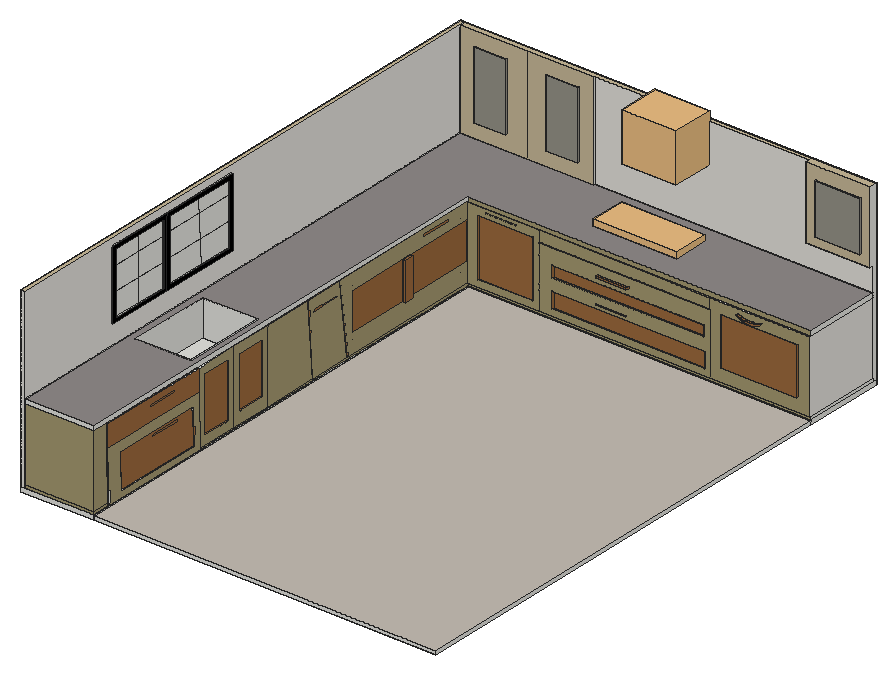
# SketchUp Ruby script. Lengths in inches.
U = 1.inch
M = Sketchup.active_model
def pt(a) = Geom::Point3d.new(a.map { |v| v * U })
def face(e, loops, mat)
  f = e.add_face(loops[0].map { |a| pt(a) })
  loops[1..].each { |l| e.add_face(l.map { |a| pt(a) }).erase! }
  f.material = f.back_material = mat if mat
  f
end
# faces: each face lists its corners as indices into pts; further lists are holes
def faces(e, pts, list, mat = nil) = list.each { |f| face(e, (f[0].is_a?(Array) ? f : [f]).map { |l| l.map { |i| pts[i] } }, mat) }
# xy, xz, yz: faces in a plane at the given z, y or x. An outline is a flat list of corners, or four numbers for a rectangle; further outlines are holes
def ring(l) = l.size == 4 ? [[l[0], l[1]], [l[2], l[1]], [l[2], l[3]], [l[0], l[3]]] : l.each_slice(2).to_a
def flat(e, list, mat, &to3) = list.each { |f| face(e, (f[0].is_a?(Array) ? f : [f]).map { |l| ring(l).map { |u, v| to3.(u, v) } }, mat) }
def xy(e, z, list, mat = nil) = flat(e, list, mat) { |x, y| [x, y, z] }
def xz(e, y, list, mat = nil) = flat(e, list, mat) { |x, z| [x, y, z] }
def yz(e, x, list, mat = nil) = flat(e, list, mat) { |y, z| [x, y, z] }
def lines(e, pts, list) = list.each { |a, b| e.add_line(pt(pts[a]), pt(pts[b])) }
# prism: a flat outline (further loops are holes) pulled along v
def prism(e, loops, v, mat = nil)
  f = face(e, loops, mat); d = Geom::Vector3d.new(v.map { |x| x * U })
  f.pushpull(f.normal.samedirection?(d) ? d.length : -d.length)
end
def box(e, o, s, mat = nil) = prism(e, [[o, [o[0] + s[0], o[1], o[2]], [o[0] + s[0], o[1] + s[1], o[2]], [o[0], o[1] + s[1], o[2]]]], [0, 0, s[2]], mat)
def at(x, y, z, deg = 0) = Geom::Transformation.translation(pt([x, y, z])) * Geom::Transformation.rotation(ORIGIN, Z_AXIS, deg.degrees)
def axes(o, x, y, z) = Geom::Transformation.new([*x, 0, *y, 0, *z, 0, *pt(o).to_a, 1])
def part(name) = M.definitions.add(name)
# library, detail: a bought-in or finely detailed component or shape, given as its bounding box
def library(name, o, s) = part(name).tap { |d| box(d.entities, o, s) }
def detail(e, o, s) = box(e.add_group.entities, o, s)
def put(e, d, t, mat = nil) = e.add_instance(d, t).tap { |i| i.material = mat if mat }
def group(e, t, mat = nil) = e.add_group.tap { |g| g.transformation = t; g.material = mat if mat }.entities
root = M.entities
M.materials.add("[Color M09]").color = [0, 0, 0]
M.materials.add("[Field Rectangle Tile]").color = [196, 189, 179]
M.materials.add("[Formica Graystone]").color = [149, 146, 135]
M.materials.add("[Marble Carrara Gold Floor Tile]").color = [225, 223, 217]
M.materials.add("[Quartz Light Brown]").color = [199, 184, 152]
M.materials.add("[Stone Marble]").color = [143, 138, 136]
M.materials.add("[Wood Floor]").color = [155, 105, 61]
M.materials.add("[Wood Lumber ButtJoined]").color = [164, 152, 112]
c1 = library("CGP650SETSS",[0,0,0],[36,20.75,4.5])
c2 = library("PV977NSS_GEProfile",[-17.9375,-27.5625,-0.25],[35.95,27.64,32.08])
xy(root,0,[[0,0,0,365.375,276.25,365.375,276.25,311.14,48.625,311.14,48.625,0],[48.625,0,276.25,311.14]])
xy(root,2.4,[[48.625,0,276.25,311.14]],"[Field Rectangle Tile]")
xy(root,3,[[0,0,3,365.375],[3,0,3,362.375,276.25,362.375,276.25,311.14,48.625,311.14,48.625,0],[3,362.375,276.25,365.375]])
xy(root,5,[[3,0,3,362.375,276.25,362.375,276.25,311.14,48.625,311.14,48.625,0],[48.625,85.77,49.625,114.5],[48.625,114.5,49.625,143.24],[48.625,143.24,48.625,310.14,48.63,310.14,49.23,210.02,48.625,210.01,48.63,208.96,49.23,208.96,49.4,181.37,48.625,181.36,48.63,180.08,49.41,180.09,49.625,143.24],[48.625,310.14,48.625,311.14,48.63,310.14],
  [48.63,310.14,48.625,311.14,96,311.14,96,310.14],[96,310.14,210.05,311.14],[210.05,310.14,276.25,311.14]])
xy(root,9.28,[[105.11,310.14,206.3,311.14]],"[Wood Floor]")
xy(root,9.41,[[55.64,310.14,92.32,311.14]],"[Wood Floor]")
xy(root,11.1,[[48.625,90.01,49.625,110.7]],"[Wood Floor]")
xy(root,12.77,[[48.625,119.14,49.625,139.2]],"[Wood Floor]")
xy(root,14.16,[[217.67,309.14,268.43,310.14]],"[Wood Floor]")
xy(root,17.5625,[[48.2,213.88,49.2,213.88,48.95,256.07,47.95,256.07],[47.95,256.07,48.95,256.07,48.91,262.51,47.91,262.51],[47.91,262.51,48.91,262.51,48.625,311.14,47.625,311.13]])
xy(root,17.5625,[[48.95,256.07,48.91,262.51,50.91,262.52,50.95,256.08]],"[Wood Floor]")
xy(root,19.85,[[105.11,310.14,206.3,311.14]])
xy(root,28.14,[[105.21,310.14,206.08,311.14]],"[Wood Floor]")
xy(root,32,[[7.71,85.84,44.64,141.53]])
xy(root,35.58,[[105.21,310.14,206.08,311.14]])
xy(root,39.34,[[135.71,308.14,155.96,310.14]])
xy(root,40.4,[[135.71,308.14,155.96,310.14]],"[Wood Floor]")
xy(root,42.88,[[48.2,213.88,47.95,256.07,48.95,256.07,49.2,213.88],[47.95,256.07,47.91,262.51,48.91,262.51,48.95,256.07],[47.91,262.51,47.625,311.13,48.625,311.14,48.91,262.51]])
xy(root,42.88,[[48.95,256.07,50.95,256.08,50.91,262.52,48.91,262.51]],"[Wood Floor]")
xy(root,45.53,[[217.67,309.14,268.43,310.14]],"[Wood Floor]")
xy(root,46.96,[[48.625,119.14,49.625,139.2]],"[Wood Floor]")
xy(root,47.72,[[55.64,310.14,92.32,311.14]])
xy(root,47.85,[[48.625,90.01,49.625,110.7]],"[Wood Floor]")
xy(root,53,[[48.625,85.77,49.625,114.5],[48.625,114.5,49.625,143.24],[48.625,143.24,49.625,143.24,49.43,176.36,48.65,176.35,48.65,177.34,49.42,177.35,49.27,202.84,48.67,202.83,48.66,203.75,49.26,203.75,48.63,310.14,48.625,310.14],[48.625,310.14,48.63,310.14,48.625,311.14]])
xy(root,53,[[210.05,310.14,276.25,311.14]],"[Marble Carrara Gold Floor Tile]")
xy(root,53,[[48.63,310.14,96,310.14,96,311.14,48.625,311.14],[96,310.14,210.05,311.14]],"[Wood Lumber ButtJoined]")
xy(root,56,[[3,361.375,47.37,362.375],[47.37,361.375,91.74,362.375]])
xy(root,56,[[[3,0,48.625,0,48.625,311.14,276.25,311.14,276.25,362.375,91.74,362.375,91.74,361.375,3,361.375],[7.71,85.84,44.64,141.53]]],"[Stone Marble]")
xy(root,65.88,[[13.14,360.375,34.2,361.375]])
xy(root,65.88,[[60.64,360.375,81.7,361.375]],"[Formica Graystone]")
xy(root,69.45,[[3,72.13,4,116.73],[3,116.73,4,171.32]])
xy(root,71.58,[[3,74.26,4,94.43],[3,94.43,4,114.6]],"[Color M09]")
xy(root,71.82,[[3,119.1,4,146.39],[3,146.39,4,168.95]],"[Color M09]")
xy(root,72.01,[[233.56,360.375,276.25,362.375]],"[Quartz Light Brown]")
xy(root,78.16,[[240.1875,359.375,270.125,360.375]],"[Formica Graystone]")
xy(root,110.69,[[13.14,360.375,34.2,361.375],[60.64,360.375,81.7,361.375]],"[Formica Graystone]")
xy(root,111.41,[[240.1875,359.375,270.125,360.375]],"[Formica Graystone]")
xy(root,112.89,[[3,119.1,4,144.03],[3,144.03,4,168.95]])
xy(root,113.13,[[3,74.26,4,94.43],[3,94.43,4,114.6]])
xy(root,115.26,[[3,72.13,4,116.73],[3,116.73,4,171.32]],"[Color M09]")
xy(root,120,[[0,0,3,365.375],[233.56,360.375,276.25,360.375,276.25,365.375,3,365.375,3,361.375,91.74,361.375,91.74,362.375,233.56,362.375]],"[Quartz Light Brown]")
xz(root,0,[[0,0,48.625,3],[48.625,0,276.25,2.4],[3,53,48.625,56]])
xz(root,0,[[0,3,3,120]],"[Marble Carrara Gold Floor Tile]")
xz(root,0,[[3,3,48.625,5],[3,5,48.625,53]],"[Wood Lumber ButtJoined]")
xz(root,10.64,[[49.625,5,50.625,5.02,49.92,38.78,48.92,38.75],[48.92,38.75,49.92,38.78,49.625,53.02,48.625,53]])
xz(root,20.09,[[49.55,8.65,49.05,32.52,50.05,32.54,50.55,8.67]],"[Wood Floor]")
xz(root,72.13,[[3,69.45,4,115.26]],"[Color M09]")
xz(root,74.26,[[3,71.58,4,87.12],[3,87.12,4,102.65],[3,102.65,4,113.13]],"[Color M09]")
xz(root,81.46,[[49.55,8.65,50.55,8.67,50.05,32.54,49.05,32.52]],"[Wood Floor]")
xz(root,85.77,[[48.625,5,49.625,5,48.92,38.75,48.625,53],[49.625,5,49.625,38.77,48.92,38.75],[49.625,5,49.625,38.77,49.92,38.78,50.625,5.02],[48.92,38.75,49.625,38.77,49.625,53,48.625,53],[49.625,38.77,49.625,53,49.92,38.78],
  [48.625,53,49.625,53.02,49.625,53]])
xz(root,85.84,[[7.71,32,44.64,56]])
xz(root,90.01,[[48.625,11.1,49.625,47.85]],"[Wood Floor]")
xz(root,110.7,[[48.625,11.1,49.625,47.85]],"[Wood Floor]")
xz(root,114.6,[[3,71.58,4,87.12],[3,87.12,4,102.65],[3,102.65,4,113.13]],"[Color M09]")
xz(root,116.73,[[3,69.45,4,115.26]])
xz(root,119.1,[[3,71.82,4,87.55],[3,87.55,4,103.27],[3,103.27,4,112.89]],"[Color M09]")
xz(root,119.14,[[48.625,12.77,49.625,46.96]],"[Wood Floor]")
xz(root,139.2,[[48.625,12.77,49.625,46.96]],"[Wood Floor]")
xz(root,141.53,[[7.71,32,44.64,56]])
xz(root,143.24,[[48.625,5,49.625,53]])
xz(root,168.95,[[3,71.82,4,87.55],[3,87.55,4,103.27],[3,103.27,4,112.89]],"[Color M09]")
xz(root,171.32,[[3,69.45,4,115.26]],"[Color M09]")
xz(root,213.88,[[48.2,17.5625,49.2,42.88]])
xz(root,256.07,[[47.95,17.5625,48.95,42.88]],"[Wood Floor]")
xz(root,262.51,[[47.91,17.5625,48.91,42.88]])
xz(root,308.14,[[135.71,23.15,155.96,24.21],[135.71,39.34,155.96,40.4],[237.21,47.2,238.71,47.28,240.19,47.52,241.65,47.91,243.05,48.46,244.39,49.15,245.64,49.98,244.29,49.48,242.91,49.08,241.5,48.76,240.08,48.53,238.64,48.4,237.21,48.35,235.77,48.4,234.33,48.53,232.91,48.76,231.5,49.08,230.12,49.48,228.77,49.98,230.02,49.15,231.36,48.46,232.76,47.91,234.22,47.52,235.7,47.28]],"[Wood Floor]")
xz(root,309.14,[[217.67,14.16,268.43,45.53]],"[Wood Floor]")
xz(root,310.14,[[96,45.7,210.05,46.01],[60.76,50.07,81.01,51.14]],"[Wood Floor]")
xz(root,310.14,[[[48.625,5,96,53],[55.64,9.41,92.32,47.72],[60.76,50.07,81.01,51.14]],[[96,5,210.05,45.7],[105.11,9.28,206.3,19.85],[105.21,28.14,206.08,35.58],[135.71,39.34,155.96,40.4]],[[210.05,5,276.25,53],[217.67,14.16,268.43,45.53],[237.21,47.2,235.7,47.28,234.22,47.52,232.76,47.91,231.36,48.46,230.02,49.15,228.77,49.98,230.12,49.48,231.5,49.08,232.91,48.76,234.33,48.53,235.77,48.4,237.21,48.35,238.64,48.4,240.08,48.53,241.5,48.76,242.91,49.08,244.29,49.48,245.64,49.98,244.39,49.15,243.05,48.46,241.65,47.91,240.19,47.52,238.71,47.28]],[96,46.01,210.05,53]],"[Wood Lumber ButtJoined]")
xz(root,311.14,[[48.625,0,276.25,2.4],[48.625,2.4,276.25,3]])
xz(root,311.14,[[105.11,9.28,206.3,19.85],[55.64,9.41,92.32,47.72],[105.21,28.14,206.08,35.58]],"[Wood Floor]")
xz(root,311.14,[[48.625,3,276.25,5],[48.625,53,276.25,56]],"[Wood Lumber ButtJoined]")
xz(root,359.375,[[240.1875,78.16,270.125,111.41]],"[Formica Graystone]")
xz(root,360.375,[[13.14,65.88,34.2,110.69],[60.64,65.88,81.7,110.69]],"[Formica Graystone]")
xz(root,360.375,[[[233.56,72.01,276.25,120],[240.1875,78.16,270.125,111.41]]],"[Quartz Light Brown]")
xz(root,361.375,[[[3,56,47.37,120],[13.14,65.88,34.2,110.69]],[[47.37,56,91.74,120],[60.64,65.88,81.7,110.69]]],"[Quartz Light Brown]")
xz(root,362.375,[[3,3,276.25,5],[3,5,276.25,53],[3,53,276.25,56]])
xz(root,362.375,[[91.74,56,276.25,56,276.25,72.01,233.56,72.01,233.56,120,91.74,120]],"[Marble Carrara Gold Floor Tile]")
xz(root,365.375,[[0,0,276.25,3],[0,3,3,120],[3,3,276.25,120]])
yz(root,0,[[0,0,365.375,3],[0,3,365.375,120]])
yz(root,3,[[0,3,362.375,5],[362.375,3,365.375,3,365.375,120,361.375,120,361.375,56,362.375,56],[0,5,362.375,53],[0,53,362.375,56],[[72.13,69.45,116.73,115.26],[74.26,71.58,114.6,113.13]],
  [[116.73,69.45,171.32,115.26],[119.1,71.82,168.95,112.89]]])
yz(root,3,[[[0,56,361.375,120],[72.13,69.45,171.32,115.26]]],"[Marble Carrara Gold Floor Tile]")
yz(root,4,[[[72.13,69.45,116.73,115.26],[74.26,71.58,114.6,113.13]],[[116.73,69.45,171.32,115.26],[119.1,71.82,168.95,112.89]]],"[Color M09]")
yz(root,7.71,[[85.84,32,141.53,56]])
yz(root,13.14,[[360.375,65.88,361.375,110.69]],"[Formica Graystone]")
yz(root,34.2,[[360.375,65.88,361.375,110.69]],"[Formica Graystone]")
yz(root,44.64,[[85.84,32,141.53,56]])
yz(root,48.625,[[0,0,311.14,2.4],[0,2.4,311.14,3],[310.14,5,311.14,17.5625],[310.14,17.5625,311.14,42.88],[310.14,42.88,311.14,53],
  [0,53,311.14,56]])
yz(root,48.625,[[143.24,5,310.14,53],[90.01,11.1,110.7,47.85],[119.14,12.77,139.2,46.96]],"[Wood Floor]")
yz(root,48.625,[[0,3,311.14,5],[0,5,85.77,53]],"[Wood Lumber ButtJoined]")
yz(root,49.625,[[[85.77,5,114.5,53],[90.01,11.1,110.7,47.85]],[[114.5,5,143.24,53],[119.14,12.77,139.2,46.96]]],"[Wood Lumber ButtJoined]")
yz(root,55.64,[[310.14,9.41,311.14,47.72]],"[Wood Floor]")
yz(root,60.64,[[360.375,65.88,361.375,110.69]],"[Formica Graystone]")
yz(root,81.7,[[360.375,65.88,361.375,110.69]],"[Formica Graystone]")
yz(root,91.74,[[361.375,56,362.375,120]])
yz(root,92.32,[[310.14,9.41,311.14,47.72]],"[Wood Floor]")
yz(root,105.11,[[310.14,9.28,311.14,19.85]],"[Wood Floor]")
yz(root,105.21,[[310.14,28.14,311.14,35.58]],"[Wood Floor]")
yz(root,135.71,[[308.14,39.34,310.14,40.4]],"[Wood Floor]")
yz(root,155.96,[[308.14,39.34,310.14,40.4]],"[Wood Floor]")
yz(root,206.08,[[310.14,28.14,311.14,35.58]],"[Wood Floor]")
yz(root,206.3,[[310.14,9.28,311.14,19.85]],"[Wood Floor]")
yz(root,217.67,[[309.14,14.16,310.14,45.53]],"[Wood Floor]")
yz(root,233.56,[[360.375,72.01,362.375,120]])
yz(root,240.1875,[[359.375,78.16,360.375,111.41]],"[Formica Graystone]")
yz(root,268.43,[[309.14,14.16,310.14,45.53]],"[Wood Floor]")
yz(root,270.125,[[359.375,78.16,360.375,111.41]],"[Formica Graystone]")
yz(root,276.25,[[0,0,311.14,2.4],[311.14,0,365.375,3],[311.14,3,362.375,5],[362.375,3,365.375,3,365.375,120,360.375,120,360.375,72.01,362.375,72.01],[311.14,53,362.375,56]])
yz(root,276.25,[[310.14,5,362.375,53]],"[Marble Carrara Gold Floor Tile]")
p = [[48.92,85.77,38.75],[49.625,85.77,5],[49.625,10.64,5],[48.92,10.64,38.75],[49.55,81.46,8.65],[49.05,81.46,32.52],
  [49.05,20.09,32.52],[49.55,20.09,8.65],[50.625,85.77,5.02],[50.625,10.64,5.02],[49.92,85.77,38.78],[49.92,10.64,38.78],
  [50.05,81.46,32.54],[50.55,81.46,8.67],[50.55,20.09,8.67],[50.05,20.09,32.54],[49.625,143.24,5],[49.41,180.09,5],
  [49.43,176.36,53],[49.625,143.24,53],[49.47,169.09,39.49],[49.47,169.09,38.43],[49.59,148.84,38.43],[49.59,148.84,39.49],
  [48.63,180.08,5],[48.625,181.36,5],[48.65,177.34,53],[48.65,176.35,53],[49.4,181.37,5],[49.42,177.35,53],
  [49.23,208.96,5],[49.27,202.84,53],[49.27,202.01,45.33],[49.27,202.01,44.26],[49.4,181.76,44.26],[49.4,181.76,45.33],
  [48.63,208.96,5],[48.625,210.01,5],[48.66,203.75,53],[48.67,202.83,53],[48.625,311.14,5],[48.625,311.14,17.5625],
  [48.91,262.51,17.5625],[48.95,256.07,17.5625],[49.2,213.88,17.5625],[49.2,213.88,42.88],[48.95,256.07,42.88],[48.91,262.51,42.88],
  [48.625,311.14,42.88],[48.625,311.14,53],[48.63,310.14,53],[49.26,203.75,53],[49.23,210.02,5],[48.63,310.14,5],
  [48.73,293.66,49.63],[48.73,293.66,48.57],[48.85,273.41,48.57],[48.85,273.41,49.63],[49.11,68.46,29.95],[49.13,68.46,28.89],
  [49.13,48.21,28.89],[49.11,48.21,29.95],[5.95,213.99,45.65],[5.95,213.99,13.83],[5.41,304.36,13.83],[5.41,304.36,45.65],
  [47.95,256.07,17.5625],[47.91,262.51,17.5625],[47.91,262.51,42.88],[47.95,256.07,42.88],[50.95,256.08,17.5625],[50.95,256.08,42.88],
  [50.91,262.52,17.5625],[50.91,262.52,42.88],[47.625,311.13,42.88],[47.625,311.13,17.5625],[48.625,10.64,53],[48.625,85.77,53],
  [49.625,85.77,38.77],[49.625,10.64,53.02],[49.625,85.77,53],[49.625,85.77,53.02],[49.72,65.33,48.42],[49.74,65.33,47.36],
  [49.74,45.08,47.36],[49.72,45.08,48.42],[235.7,310.14,47.28],[237.21,310.14,47.2],[237.21,308.14,47.2],[235.7,308.14,47.28],
  [238.71,310.14,47.28],[238.71,308.14,47.28],[234.22,310.14,47.52],[234.22,308.14,47.52],[240.19,310.14,47.52],[240.19,308.14,47.52],
  [232.76,310.14,47.91],[232.76,308.14,47.91],[241.65,310.14,47.91],[241.65,308.14,47.91],[231.36,310.14,48.46],[231.36,308.14,48.46],
  [243.05,310.14,48.46],[243.05,308.14,48.46],[235.77,310.14,48.4],[234.33,310.14,48.53],[234.33,308.14,48.53],[235.77,308.14,48.4],
  [237.21,310.14,48.35],[237.21,308.14,48.35],[238.64,310.14,48.4],[238.64,308.14,48.4],[240.08,310.14,48.53],[240.08,308.14,48.53],
  [230.02,310.14,49.15],[230.02,308.14,49.15],[232.91,310.14,48.76],[232.91,308.14,48.76],[241.5,310.14,48.76],[241.5,308.14,48.76],
  [244.39,310.14,49.15],[244.39,308.14,49.15],[231.5,310.14,49.08],[231.5,308.14,49.08],[242.91,310.14,49.08],[242.91,308.14,49.08],
  [228.77,310.14,49.98],[228.77,308.14,49.98],[230.12,310.14,49.48],[230.12,308.14,49.48],[244.29,310.14,49.48],[244.29,308.14,49.48],
  [245.64,310.14,49.98],[245.64,308.14,49.98],[347.17,609.45,0],[347.17,609.45,-0.8125],[49.2,214.25,13.83],[49.2,214.25,45.65],
  [48.66,304.62,13.83],[48.66,304.62,45.65],[3,94.43,111.375],[3,94.43,102.65],[3,94.43,113.13],[3,74.26,102.65],
  [3,94.43,87.12],[3,114.6,102.65],[3,74.26,87.12],[3,94.43,71.58],[3,114.6,87.12],[3,144.03,112.89],
  [3,144.58,103.27],[3,119.1,103.27],[3,145.49,87.55],[3,168.95,103.27],[3,119.1,87.55],[3,146.39,71.82],
  [3,168.95,87.55]]
faces(root,p,[[[0,1,2,3],[4,5,6,7]],[2,1,8,9],[62,63,64,65],[66,67,68,69],[43,46,47,42],[41,48,74,75],[3,76,77,0],[0,3,11,10,78],
  [86,87,88,89],[87,90,91,88],[92,86,89,93],[90,94,95,91],[96,92,93,97],[94,98,99,95],[100,96,97,101],[98,102,103,99],
  [114,100,101,115],[102,120,121,103],[126,114,115,127],[120,132,133,121],[77,76,79,81]])
faces(root,p,[[[8,10,11,9],[12,13,14,15]],[[16,17,18,19],[20,21,22,23]],[[28,30,31,29],[32,33,34,35]],[[40,41,42,43,44,45,46,47,48,49,50,51,52,53],[54,55,56,57]]],"[Wood Lumber ButtJoined]")
faces(root,p,[[24,25,26,27],[18,17,24,27],[28,29,26,25],[36,37,38,39],[31,30,36,39],[52,51,38,37],[[4,5,6,7],[58,59,60,61]],[4,7,14,13],
  [46,43,70,71],[71,70,72,73],[42,47,73,72],[61,60,59,58],[6,5,12,15],[23,22,21,20],[[79,11,10,80,81],[82,83,84,85]],[35,34,33,32],
  [85,84,83,82],[104,105,106,107],[108,104,107,109],[110,108,109,111],[112,110,111,113],[105,116,117,106],[118,112,113,119],[57,56,55,54],
  [116,122,123,117],[124,118,119,125],[122,128,129,123],[130,124,125,131],[128,126,127,129],[132,130,131,133]],"[Wood Floor]")
lines(root,p,[[134,135],[136,63],[137,62],[138,64],[139,65],[140,141],[142,140],[143,141],[141,144],[141,145],[146,144],[144,147],
  [144,148],[149,150],[151,150],[150,152],[150,153],[154,152],[152,155],[152,156]])
put(root,c1,axes([118.51,327.51,56],[1.54088,0,0],[0,1.133,0],[0,0,0.87241]))
put(root,c2,at(149.68,362.375,94.61))
